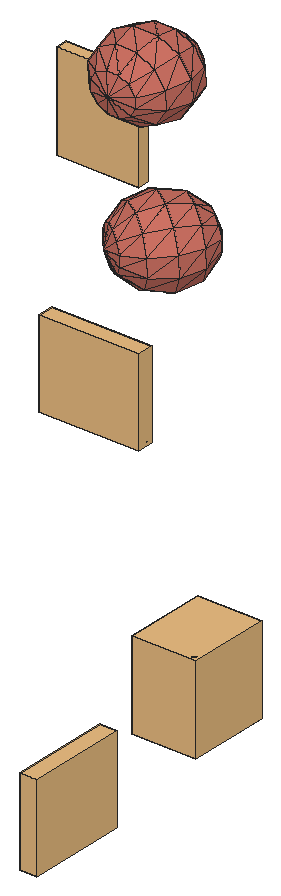
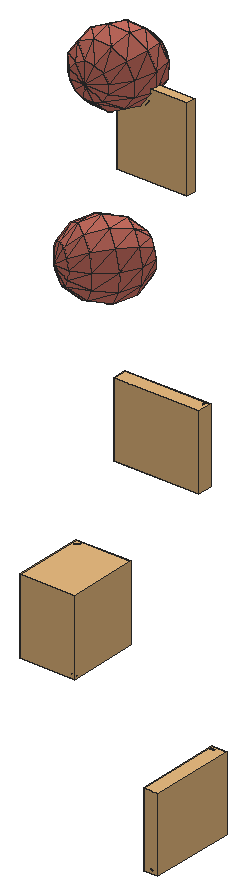
# SketchUp Ruby script. Lengths in inches.
U = 1.inch
M = Sketchup.active_model
def pt(a) = Geom::Point3d.new(a.map { |v| v * U })
def face(e, loops, mat)
  f = e.add_face(loops[0].map { |a| pt(a) })
  loops[1..].each { |l| e.add_face(l.map { |a| pt(a) }).erase! }
  f.material = f.back_material = mat if mat
  f
end
# faces: each face lists its corners as indices into pts; further lists are holes
def faces(e, pts, list, mat = nil) = list.each { |f| face(e, (f[0].is_a?(Array) ? f : [f]).map { |l| l.map { |i| pts[i] } }, mat) }
# xy, xz, yz: faces in a plane at the given z, y or x. An outline is a flat list of corners, or four numbers for a rectangle; further outlines are holes
def ring(l) = l.size == 4 ? [[l[0], l[1]], [l[2], l[1]], [l[2], l[3]], [l[0], l[3]]] : l.each_slice(2).to_a
def flat(e, list, mat, &to3) = list.each { |f| face(e, (f[0].is_a?(Array) ? f : [f]).map { |l| ring(l).map { |u, v| to3.(u, v) } }, mat) }
def xy(e, z, list, mat = nil) = flat(e, list, mat) { |x, y| [x, y, z] }
def xz(e, y, list, mat = nil) = flat(e, list, mat) { |x, z| [x, y, z] }
def yz(e, x, list, mat = nil) = flat(e, list, mat) { |y, z| [x, y, z] }
def lines(e, pts, list) = list.each { |a, b| e.add_line(pt(pts[a]), pt(pts[b])) }
# prism: a flat outline (further loops are holes) pulled along v
def prism(e, loops, v, mat = nil)
  f = face(e, loops, mat); d = Geom::Vector3d.new(v.map { |x| x * U })
  f.pushpull(f.normal.samedirection?(d) ? d.length : -d.length)
end
def box(e, o, s, mat = nil) = prism(e, [[o, [o[0] + s[0], o[1], o[2]], [o[0] + s[0], o[1] + s[1], o[2]], [o[0], o[1] + s[1], o[2]]]], [0, 0, s[2]], mat)
def at(x, y, z, deg = 0) = Geom::Transformation.translation(pt([x, y, z])) * Geom::Transformation.rotation(ORIGIN, Z_AXIS, deg.degrees)
def axes(o, x, y, z) = Geom::Transformation.new([*x, 0, *y, 0, *z, 0, *pt(o).to_a, 1])
def part(name) = M.definitions.add(name)
# library, detail: a bought-in or finely detailed component or shape, given as its bounding box
def library(name, o, s) = part(name).tap { |d| box(d.entities, o, s) }
def detail(e, o, s) = box(e.add_group.entities, o, s)
def put(e, d, t, mat = nil) = e.add_instance(d, t).tap { |i| i.material = mat if mat }
def group(e, t, mat = nil) = e.add_group.tap { |g| g.transformation = t; g.material = mat if mat }.entities
root = M.entities
M.materials.add("green").color = [174, 139, 102]
M.materials.add("vio").color = [206, 114, 100]
c1 = part("3DGeom~247_Defintion")
p = [[-255.5,94.92,-415.28],[-6.35,103.625,-485.08],[-12.59,-116.1,-481.02],[239.09,-105.72,-421.38],[244.5,84.5625,-424.9],[1.59,295.58,-359.16],
  [-248.62,261.16,-306.23],[-255.5,94.92,-415.28],[-248.62,261.16,-306.23],[-260.91,-95.36,-411.76],[-15.46,-304.71,-348.07],[236.61,-269.07,-306.25],
  [-255.5,94.92,-415.28],[-260.91,-95.36,-411.76],[426.72,-67.02,-248.84],[429.84,42.84,-250.87],[426.72,-67.02,-248.84],[251.38,250.8,-315.85],
  [429.84,42.84,-250.87],[244.5,84.5625,-424.9],[251.38,250.8,-315.85],[239.09,-105.72,-421.38],[425.28,-161.33,-182.37],[236.61,-269.07,-306.25],
  [239.09,-105.72,-421.38],[426.72,-67.02,-248.84],[-436.1875,60.78,-234.21],[-255.5,94.92,-415.28],[-260.91,-95.36,-411.76],[-432.22,156.76,-171.25],
  [-248.62,261.16,-306.23],[-260.91,-95.36,-411.76],[-263.39,-258.71,-296.63],[-439.31,-49.07,-232.18],[-263.39,-258.71,-296.63],[9.11,408.34,-137.01],
  [251.38,250.8,-315.85],[1.59,295.58,-359.16],[-242.11,358.81,-113.84],[1.59,295.58,-359.16],[-248.62,261.16,-306.23],[-242.11,358.81,-113.84],
  [1.59,295.58,-359.16],[-263.39,-258.71,-296.63],[-15.46,-304.71,-348.07],[-14.18,-411.68,-121.86],[-15.46,-304.71,-348.07],[237.72,-361.7,-110.34],
  [-15.46,-304.71,-348.07],[236.61,-269.07,-306.25],[251.38,250.8,-315.85],[433.81,138.82,-187.91],[429.84,42.84,-250.87],[257.89,348.45,-123.46],
  [251.38,250.8,-315.85],[257.89,348.45,-123.46],[251.38,250.8,-315.85],[236.61,-269.07,-306.25],[425.92,-214.8125,-69.26],[237.72,-361.7,-110.34],
  [236.61,-269.07,-306.25],[-428.46,213.14,-60.17],[-242.11,358.81,-113.84],[-263.39,-258.71,-296.63],[-262.28,-351.34,-100.72],[-440.74,-143.38,-165.7],
  [-262.28,-351.34,-100.72],[429.84,42.84,-250.87],[500,-10.36,-9.62],[429.84,42.84,-250.87],[-500,10.36,9.62],[437.57,195.19,-76.83],
  [257.89,348.45,-123.46],[-440.1,-196.87,-52.6],[14.18,411.68,121.86],[-237.72,361.7,110.34],[-242.11,358.81,-113.84],[-237.72,361.7,110.34],
  [262.28,351.34,100.72],[257.89,348.45,-123.46],[262.28,351.34,100.72],[-262.28,-351.34,-100.72],[-9.11,-408.34,137.01],[242.11,-358.81,113.84],
  [-425.92,214.8125,69.26],[-237.72,361.7,110.34],[237.72,-361.7,-110.34],[428.46,-213.14,60.17],[237.72,-361.7,-110.34],[242.11,-358.81,113.84],
  [-262.28,-351.34,-100.72],[-257.89,-348.45,123.46],[-257.89,-348.45,123.46],[440.1,196.87,52.6],[262.28,351.34,100.72],[-437.57,-195.19,76.83],
  [432.22,-156.76,171.25],[436.1875,-60.78,234.21],[439.31,49.07,232.18],[440.74,143.38,165.7],[-433.81,-138.82,187.91],[-429.84,-42.84,250.87],
  [-426.72,67.02,248.84],[-425.28,161.33,182.37],[263.39,258.71,296.63],[263.39,258.71,296.63],[262.28,351.34,100.72],[242.11,-358.81,113.84],
  [-251.38,-250.8,315.85],[15.46,304.71,348.07],[263.39,258.71,296.63],[-236.61,269.07,306.25],[-236.61,269.07,306.25],[-237.72,361.7,110.34],
  [248.62,-261.16,306.23],[242.11,-358.81,113.84],[248.62,-261.16,306.23],[-236.61,269.07,306.25],[-257.89,-348.45,123.46],[-1.59,-295.58,359.16],
  [-257.89,-348.45,123.46],[-1.59,-295.58,359.16],[-251.38,-250.8,315.85],[248.62,-261.16,306.23],[-1.59,-295.58,359.16],[260.91,95.36,411.76],
  [260.91,95.36,411.76],[263.39,258.71,296.63],[248.62,-261.16,306.23],[-244.5,-84.5625,424.9],[-244.5,-84.5625,424.9],[255.5,-94.92,415.28],
  [255.5,-94.92,415.28],[260.91,95.36,411.76],[248.62,-261.16,306.23],[255.5,-94.92,415.28],[-429.84,-42.84,250.87],[-239.09,105.73,421.38],
  [-426.72,67.02,248.84],[-239.09,105.73,421.38],[-429.84,-42.84,250.87],[-244.5,-84.5625,424.9],[-239.09,105.73,421.38],[12.59,116.1,481.02],
  [260.91,95.36,411.76],[263.39,258.71,296.63],[263.39,258.71,296.63],[15.46,304.71,348.07],[-1.59,-295.58,359.16],[248.62,-261.16,306.23],
  [255.5,-94.92,415.28],[-239.09,105.73,421.38],[15.46,304.71,348.07],[-236.61,269.07,306.25],[-251.38,-250.8,315.85],[6.35,-103.625,485.08],
  [-251.38,-250.8,315.85],[-239.09,105.73,421.38],[15.46,304.71,348.07],[-239.09,105.73,421.38]]
faces(c1.entities,p,[[0,1,2],[1,3,2],[1,4,3],[5,4,1],[6,1,7],[8,5,1],[9,2,10],[2,11,10],
  [2,3,11],[12,2,13],[4,14,3],[4,15,16],[17,18,19],[5,20,4],[21,22,23],[24,25,22],
  [26,27,28],[29,27,26],[29,30,27],[31,10,32],[33,28,34],[26,28,33],[35,36,37],[38,39,40],
  [41,35,42],[43,44,45],[46,47,45],[48,49,47],[50,51,52],[53,51,54],[35,55,56],[57,58,59],
  [60,22,58],[61,30,29],[61,62,30],[63,45,64],[65,34,66],[33,34,65],[25,67,68],[69,51,68],
  [22,25,68],[26,33,70],[29,26,70],[33,65,70],[51,71,68],[72,71,51],[58,22,68],[61,29,70],
  [65,66,73],[65,73,70],[74,55,35],[75,35,76],[77,74,35],[78,71,79],[74,80,55],[81,45,82],
  [45,47,83],[45,83,82],[84,62,61],[84,85,62],[86,58,87],[88,87,89],[90,82,91],[73,66,92],
  [71,93,68],[94,93,71],[87,58,68],[84,61,70],[73,92,95],[73,95,70],[96,87,68],[97,96,68],
  [98,97,68],[99,98,68],[93,99,68],[95,100,70],[100,101,70],[101,102,70],[103,84,70],[102,103,70],
  [104,99,93],[105,93,106],[107,87,96],[103,85,84],[95,92,108],[95,108,100],[109,110,80],[109,80,74],
  [103,111,85],[112,74,113],[82,83,114],[115,96,116],[117,109,74],[118,82,119],[120,121,122],[82,123,124],
  [125,98,99],[126,99,127],[128,96,97],[102,111,103],[100,108,129],[100,130,101],[131,97,98],[132,98,133],
  [134,97,135],[136,137,138],[102,139,111],[140,141,142],[143,144,145],[143,146,147],[148,149,150],[151,152,153],
  [154,148,155],[156,155,141],[157,143,158],[148,150,155],[155,150,144],[155,144,143],[141,143,159],[141,155,143]],"vio")
c2 = library("3DGeom~179_Defintion",[-58.28,-500,-420.6],[116.56,1000,841.2])
c3 = part("3DGeom~180_Defintion")
p = [[-21.41,-458.84,-420.6],[-21.53,-500,-365.15],[-53.32,-468.47,-406.125],[10.44,-469.79,-407.35],[-21.53,-500,-365.15],[10.44,-469.79,-407.35],
  [-3.01,-461.98,-417.24],[-53.32,-468.47,-406.125],[-39.83,-461.21,-416.53],[10.38,-490.37,-379.625],[-21.53,-500,-365.15],[10.44,-469.79,-407.35],
  [10.38,-490.37,-379.625],[10.44,-469.79,-407.35],[15.34,-480.18,-393.58],[-53.32,-468.47,-406.125],[-21.53,-500,-365.15],[-53.38,-489.05,-378.4],
  [-53.32,-468.47,-406.125],[-53.38,-489.05,-378.4],[-58.28,-478.66,-392.17],[-21.53,-500,-365.15],[10.38,-490.37,-379.625],[-3.11,-497.625,-369.22],
  [-21.53,-500,-365.15],[-39.93,-496.86,-368.51],[-53.38,-489.05,-378.4],[21.98,487.39,420.6],[20.96,500,348.46],[2.62,499.54,353.65],
  [21.98,487.39,420.6],[39.43,498.77,352.9375],[20.96,500,348.46],[21.98,487.39,420.6],[53.09,496.1875,365.88],[39.43,498.77,352.9375],
  [21.98,487.39,420.6],[2.62,499.54,353.65],[-10.67,497.51,367.11],[21.98,487.39,420.6],[58.28,492.93,383.82],[53.09,496.1875,365.88],
  [21.98,487.39,420.6],[-10.67,497.51,367.11],[-15.34,494.46,385.24],[21.98,487.39,420.6],[53.61,489.88,401.95],[58.28,492.93,383.82],
  [21.98,487.39,420.6],[-15.34,494.46,385.24],[-10.15,491.2,403.18],[21.98,487.39,420.6],[40.32,487.85,415.41],[53.61,489.88,401.95],
  [21.98,487.39,420.6],[-10.15,491.2,403.18],[3.51,488.61,416.12]]
faces(c3.entities,p,[[0,1,2],[3,4,0],[5,0,6],[0,7,8],[9,10,11],[12,13,14],[15,16,17],[18,19,20],
  [21,22,23],[24,25,26],[27,28,29],[30,31,32],[33,34,35],[36,37,38],[39,40,41],[42,43,44],
  [45,46,47],[48,49,50],[51,52,53],[54,55,56]],"green")
c4 = part("3DGeom~217_Defintion")
p = [[-278.9,104.85,-403.93],[-34.22,85.5625,-494.84],[-36.78,-106.97,-488.84],[218.15,-67.8125,-449.7],[219.62,43.35,-453.16],[33.05,253.77,-407.11],
  [-201.22,299.08,-302.625],[-278.9,104.85,-403.93],[-201.22,299.08,-302.625],[-281.85,-117.47,-397],[26.0625,-272.25,-390.72],[254.43,-163.24,-393.05],
  [-278.9,104.85,-403.93],[-281.85,-117.47,-397],[414.62,-10.48,-290.0625],[258.46,140.46,-402.51],[147.02,352.57,-249.16],[-69.62,413.17,-120.23],
  [33.05,253.77,-407.11],[-201.22,299.08,-302.625],[147.02,352.57,-249.16],[33.05,253.77,-407.11],[-448.85,96.04,-204.78],[-278.9,104.85,-403.93],
  [-281.85,-117.47,-397],[-381.57,264.25,-117.05],[-201.22,299.08,-302.625],[258.46,140.46,-402.51],[324.26,197.5,-311.32],[414.62,-10.48,-290.0625],
  [147.02,352.57,-249.16],[324.26,197.5,-311.32],[-451.4,-96.49,-198.78],[-209.29,-308.32,-283.69],[-281.85,-117.47,-397],[-209.29,-308.32,-283.69],
  [318.75,-217.36,-298.39],[318.75,-217.36,-298.39],[254.43,-163.24,-393.05],[414.62,-10.48,-290.0625],[-209.29,-308.32,-283.69],[26.0625,-272.25,-390.72],
  [137.48,-365.99,-226.76],[318.75,-217.36,-298.39],[137.48,-365.99,-226.76],[324.26,197.5,-311.32],[399.39,199.2,-204.01],[414.62,-10.48,-290.0625],
  [277.14,355.5,-63.3],[324.26,197.5,-311.32],[399.39,199.2,-204.01],[324.26,197.5,-311.32],[-267.6,363.06,40.9],[-201.22,299.08,-302.625],
  [-381.57,264.25,-117.05],[-267.6,363.06,40.9],[-201.22,299.08,-302.625],[318.75,-217.36,-298.39],[393.88,-215.66,-191.08],[393.88,-215.66,-191.08],
  [318.75,-217.36,-298.39],[414.62,-10.48,-290.0625],[459.68,-158.62,-99.89],[414.62,-10.48,-290.0625],[498.52,-61.5,-49.24],[414.62,-10.48,-290.0625],
  [500,49.66,-52.7],[414.62,-10.48,-290.0625],[399.39,199.2,-204.01],[463.72,145.08,-109.35],[414.62,-10.48,-290.0625],[414.62,-10.48,-290.0625],
  [-388.56,-261.77,-100.65],[-209.29,-308.32,-283.69],[-80.64,-416.55,-94.37],[-209.29,-308.32,-283.69],[-388.56,-261.77,-100.65],[80.64,416.55,94.37],
  [267.6,-363.06,-40.9],[393.88,-215.66,-191.08],[-498.52,61.5,49.24],[-459.68,158.62,99.89],[388.56,261.77,100.65],[399.39,199.2,-204.01],
  [388.56,261.77,100.65],[399.39,199.2,-204.01],[277.14,355.5,-63.3],[-500,-49.66,52.7],[267.6,-363.06,-40.9],[-137.48,365.99,226.76],
  [-267.6,363.06,40.9],[-393.88,215.66,191.08],[-267.6,363.06,40.9],[451.4,96.49,198.78],[388.56,261.77,100.65],[-388.56,-261.77,-100.65],
  [-277.14,-355.5,63.3],[-463.72,-145.08,109.35],[-277.14,-355.5,63.3],[267.6,-363.06,-40.9],[381.57,-264.25,117.05],[69.62,-413.17,120.23],
  [209.29,308.32,283.69],[388.56,261.77,100.65],[448.85,-96.04,204.78],[381.57,-264.25,117.05],[-318.75,217.36,298.39],[-267.6,363.06,40.9],
  [-393.88,215.66,191.08],[-318.75,217.36,298.39],[-267.6,363.06,40.9],[-414.62,10.48,290.0625],[-147.02,-352.57,249.16],[-277.14,-355.5,63.3],
  [-399.39,-199.2,204.01],[-399.39,-199.2,204.01],[-147.02,-352.57,249.16],[-26.0625,272.25,390.72],[-26.0625,272.25,390.72],[281.85,117.47,397],
  [388.56,261.77,100.65],[281.85,117.47,397],[388.56,261.77,100.65],[209.29,308.32,283.69],[381.57,-264.25,117.05],[201.22,-299.08,302.625],
  [201.22,-299.08,302.625],[-147.02,-352.57,249.16],[201.22,-299.08,302.625],[-318.75,217.36,298.39],[278.9,-104.85,403.93],[278.9,-104.85,403.93],
  [281.85,117.47,397],[-399.39,-199.2,204.01],[-147.02,-352.57,249.16],[-324.26,-197.5,311.32],[-324.26,-197.5,311.32],[201.22,-299.08,302.625],
  [278.9,-104.85,403.93],[-254.43,163.24,393.05],[-137.48,365.99,226.76],[-318.75,217.36,298.39],[-254.43,163.24,393.05],[-26.0625,272.25,390.72],
  [-137.48,365.99,226.76],[-324.26,-197.5,311.32],[-147.02,-352.57,249.16],[-33.05,-253.77,407.11],[-147.02,-352.57,249.16],[201.22,-299.08,302.625],
  [-33.05,-253.77,407.11],[36.78,106.98,488.84],[209.29,308.32,283.69],[281.85,117.47,397],[209.29,308.32,283.69],[-258.46,-140.46,402.51],
  [-258.46,-140.46,402.51],[-219.62,-43.35,453.16],[-414.62,10.48,290.0625],[-218.15,67.8125,449.7],[-414.62,10.48,290.0625],[-254.43,163.24,393.05],
  [-254.43,163.24,393.05],[-414.62,10.48,290.0625],[201.22,-299.08,302.625],[278.9,-104.85,403.93],[-324.26,-197.5,311.32],[-254.43,163.24,393.05],
  [34.22,-85.5625,494.84]]
faces(c4.entities,p,[[0,1,2],[1,3,2],[1,4,3],[5,4,1],[6,1,7],[8,5,1],[9,2,10],[2,11,10],
  [2,3,11],[12,2,13],[3,4,14],[4,15,14],[5,15,4],[11,3,14],[16,15,5],[17,18,19],
  [17,20,21],[22,23,24],[25,23,22],[25,26,23],[27,28,29],[30,31,15],[32,24,33],[34,10,35],
  [22,24,32],[10,11,36],[37,38,39],[40,41,42],[10,43,44],[45,46,47],[48,49,20],[48,50,51],
  [52,53,54],[55,17,56],[42,57,58],[59,60,61],[62,59,63],[64,62,65],[66,64,67],[68,69,70],
  [69,66,71],[72,73,74],[75,42,74],[32,33,76],[77,20,17],[77,48,20],[74,42,78],[42,79,78],
  [80,22,32],[81,22,80],[81,25,22],[82,69,83],[84,85,86],[87,32,76],[80,32,87],[88,59,62],
  [89,17,90],[89,77,17],[91,25,81],[91,92,25],[93,66,69],[93,69,94],[95,74,96],[97,76,98],
  [87,76,97],[99,62,100],[100,62,64],[96,74,101],[74,78,101],[102,103,48],[102,48,77],[104,64,66],
  [104,66,93],[100,64,104],[101,78,105],[106,107,108],[109,89,110],[80,87,111],[81,80,111],[87,97,111],
  [96,101,112],[97,113,114],[115,96,116],[117,77,89],[118,102,77],[91,81,111],[119,93,120],[121,122,123],
  [97,114,111],[101,124,125],[126,100,104],[127,101,128],[129,91,111],[130,104,93],[131,93,132],[133,134,135],
  [114,136,111],[137,104,138],[139,140,141],[142,143,144],[145,146,147],[148,149,150],[151,152,143],[151,153,154],
  [136,155,111],[156,157,158],[157,159,160],[161,129,111],[159,162,163],[147,164,165],[166,147,156],[159,143,167],
  [159,151,143],[168,165,153],[168,153,151],[156,147,168],[156,168,157],[147,165,168],[157,151,159],[157,168,151]],"vio")
c5 = library("3DGeom~175_Defintion",[-468.83,-500,-365.63],[937.66,1000,731.26])
c6 = part("3DGeom~176_Defintion")
p = [[-400.83,-477.04,-357.55],[-432.9,-455.37,-364.27],[-414.5,-464.73,-365.63],[-400.83,-477.04,-357.55],[-463.57,-474.42,-303.18],[-432.9,-455.37,-364.27],
  [-432.9,-455.37,-364.27],[-463.57,-474.42,-303.18],[-464.27,-454.05,-337.08],[-432.9,-455.37,-364.27],[-464.27,-454.05,-337.08],[-451.12,-451.46,-353.82],
  [-400.14,-497.41,-323.65],[-463.57,-474.42,-303.18],[-400.83,-477.04,-357.55],[-400.14,-497.41,-323.65],[-400.83,-477.04,-357.55],[-395.58,-489,-342.18],
  [-463.57,-474.42,-303.18],[-468.83,-462.46,-318.55],[-464.27,-454.05,-337.08],[-431.5,-496.09,-296.46],[-400.14,-497.41,-323.65],[-413.29,-500,-306.91],
  [-431.5,-496.09,-296.46],[-463.57,-474.42,-303.18],[-400.14,-497.41,-323.65],[-463.57,-474.42,-303.18],[-431.5,-496.09,-296.46],[-449.91,-486.73,-295.09],
  [426,485.85,358.46],[461.26,458.37,290.55],[449.4375,472.35,283.375],[426,485.85,358.46],[449.4375,472.35,283.375],[436.0625,486.26,287.22],
  [426,485.85,358.46],[436.0625,486.26,287.22],[424.71,496.38,301.05],[426,485.85,358.46],[468.35,448.07,306.83],[461.26,458.37,290.55],
  [426,485.85,358.46],[424.71,496.38,301.05],[418.43,500,321.17],[426,485.85,358.46],[468.83,444.22,327.84],[468.35,448.07,306.83],
  [426,485.85,358.46],[418.43,500,321.17],[418.9,496.14,342.18],[426,485.85,358.46],[462.55,447.84,347.96],[468.83,444.22,327.84],
  [426,485.85,358.46],[451.2,457.96,361.79],[462.55,447.84,347.96],[426,485.85,358.46],[437.82,471.87,365.63],[451.2,457.96,361.79]]
faces(c6.entities,p,[[0,1,2],[3,4,5],[6,7,8],[9,10,11],[12,13,14],[15,16,17],[18,19,20],[21,22,23],
  [24,25,26],[27,28,29],[30,31,32],[33,34,35],[36,37,38],[39,40,41],[42,43,44],[45,46,47],
  [48,49,50],[51,52,53],[54,55,56],[57,58,59]],"green")
c7 = library("3DGeom~167_Defintion",[-82.54,-434.125,-500],[165.09,868.26,1000])
c8 = part("3DGeom~168_Defintion")
p = [[25.15,421.84,-478.96],[-0.29,388.84,-500],[-17.78,385.7,-494.64],[25.15,421.84,-478.96],[15.1875,397.625,-498.65],[-0.29,388.84,-500],
  [25.15,421.84,-478.96],[24.5,409.7,-490.95],[25.15,421.84,-478.96],[-17.78,385.7,-494.64],[-32.61,389.04,-484],[25.15,421.84,-478.96],
  [-32.61,389.04,-484],[-40.79,397.98,-470.93],[25.15,421.84,-478.96],[-40.79,397.98,-470.93],[-40.14,410.12,-458.94],[25.15,421.84,-478.96],
  [-40.14,410.12,-458.94],[-30.83,422.2,-451.24],[25.15,421.84,-478.96],[-30.83,422.2,-451.24],[-15.35,430.99,-449.89],[25.15,421.84,-478.96],
  [-15.35,430.99,-449.89],[2.14,434.13,-455.26],[25.15,421.84,-478.96],[2.14,434.13,-455.26],[16.97,430.78,-465.89],[-23.73,-430.73,456.61],
  [-58.59,-431.87,447.46],[-40.15,-434.125,448.67],[-58.59,-431.87,447.46],[-12.82,-411.91,482.88],[-82.54,-414.19,464.58],[-58.59,-431.87,447.46],
  [-82.54,-414.19,464.58],[-74.11,-424.57,453.28],[-23.73,-430.73,456.61],[-12.82,-411.91,482.88],[-58.59,-431.87,447.46],[-12.82,-411.91,482.88],
  [-23.73,-430.73,456.61],[-13.73,-422.6,469.125],[-82.54,-414.19,464.58],[-12.82,-411.91,482.88],[-71.64,-395.37,490.85],[-82.54,-414.19,464.58],
  [-81.64,-403.5,478.33],[-12.82,-411.91,482.88],[-36.78,-394.23,500],[-12.82,-411.91,482.88],[-21.26,-401.53,494.18],[-55.22,-391.98,498.78]]
faces(c8.entities,p,[[0,1,2],[3,4,5],[6,7,4],[8,9,10],[11,12,13],[14,15,16],[17,18,19],[20,21,22],
  [23,24,25],[26,27,28],[29,30,31],[32,33,34],[35,36,37],[38,39,40],[41,42,43],[44,45,46],
  [47,46,48],[46,49,50],[51,52,50],[46,50,53]],"green")
c9 = library("3DGeom~88_Defintion",[-500,-434.28,-85.45],[1000,868.56,170.9])
c10 = part("3DGeom~89_Defintion")
p = [[-447.25,-432.03,-61.34],[-483.08,-412.0625,-15.87],[-464.16,-414.34,-85.45],[-447.25,-432.03,-61.34],[-464.16,-414.34,-85.45],[-452.93,-424.73,-76.91],
  [-464.16,-414.34,-85.45],[-483.08,-412.0625,-15.87],[-490.54,-395.51,-74.77],[-464.16,-414.34,-85.45],[-477.93,-403.65,-84.67],[-483.08,-412.0625,-15.87],
  [-500,-394.375,-39.98],[-498.62,-392.12,-58.41],[-456.71,-430.89,-26.55],[-447.25,-432.03,-61.34],[-448.63,-434.28,-42.9],[-456.71,-430.89,-26.55],
  [-483.08,-412.0625,-15.87],[-447.25,-432.03,-61.34],[-483.08,-412.0625,-15.87],[-494.3125,-401.67,-24.41],[478.73,421.99,30.62],[484.28,389.18,-27.12],
  [471.28,398.13,-35.42],[478.73,421.99,30.62],[471.28,398.13,-35.42],[459.28,410.27,-34.875],[478.73,421.99,30.62],[459.28,410.27,-34.875],
  [451.5,422.35,-25.63],[478.73,421.99,30.62],[494.79,385.84,-12.2],[484.28,389.18,-27.12],[-483.08,-412.0625,-15.87],[-456.71,-430.89,-26.55],
  [-469.32,-422.76,-16.65],[478.73,421.99,30.62],[451.5,422.35,-25.63],[450.01,431.14,-10.16],[478.73,421.99,30.62],[500,388.98,5.35],
  [494.79,385.84,-12.2],[478.73,421.99,30.62],[450.01,431.14,-10.16],[455.22,434.28,7.39],[478.73,421.99,30.62],[498.51,397.77,20.82],
  [500,388.98,5.35],[478.73,421.99,30.62],[455.22,434.28,7.39],[465.73,430.9375,22.3125],[478.73,421.99,30.62],[490.73,409.85,30.07]]
faces(c10.entities,p,[[0,1,2],[3,4,5],[6,7,8],[9,8,10],[8,11,12],[8,12,13],[14,15,16],[17,18,19],
  [20,21,12],[22,23,24],[25,26,27],[28,29,30],[31,32,33],[34,35,36],[37,38,39],[40,41,42],
  [43,44,45],[46,47,48],[49,50,51],[52,53,47]],"green")
g1 = group(root,at(15.3125,134.49,26.21))
put(g1,c1,axes([-0.78,-0.43,13.33],[0,0.00039,0],[0,0,-0.00039],[-0.00039,0,0]),"vio")
g2 = group(root,at(15.3125,134.49,26.21))
put(g2,c2,axes([-0.97,-0.42,13.11],[0,0.0004,0],[0,0,-0.0004],[-0.0004,0,0]),"green")
put(g2,c3,axes([-0.97,-0.42,13.11],[0,0.0004,0],[0,0,-0.0004],[-0.0004,0,0]),"green")
g3 = group(root,at(15.3125,134.49,26.21))
put(g3,c4,axes([-0.86,-0.25,12.61],[0,0.00039,0],[0,0,-0.00039],[-0.00039,0,0]),"vio")
g4 = group(root,at(15.3125,134.49,26.21))
put(g4,c5,axes([-0.72,-0.25,11.05],[0,0.00036,0],[0,0,-0.00036],[-0.00036,0,0]),"green")
put(g4,c6,axes([-0.72,-0.25,11.05],[0,0.00036,0],[0,0,-0.00036],[-0.00036,0,0]),"green")
g5 = group(root,at(15.3125,134.49,26.21))
put(g5,c7,axes([-1.16,-0.22,11.98],[0,0.00041,0],[0,0,-0.00041],[-0.00041,0,0]),"green")
put(g5,c8,axes([-1.16,-0.22,11.98],[0,0.00041,0],[0,0,-0.00041],[-0.00041,0,0]),"green")
g6 = group(root,at(15.3125,134.49,26.21))
put(g6,c9,axes([-1.27,-0.22,10.39],[0,0.00041,0],[0,0,-0.00041],[-0.00041,0,0]),"green")
put(g6,c10,axes([-1.27,-0.22,10.39],[0,0.00041,0],[0,0,-0.00041],[-0.00041,0,0]),"green")
